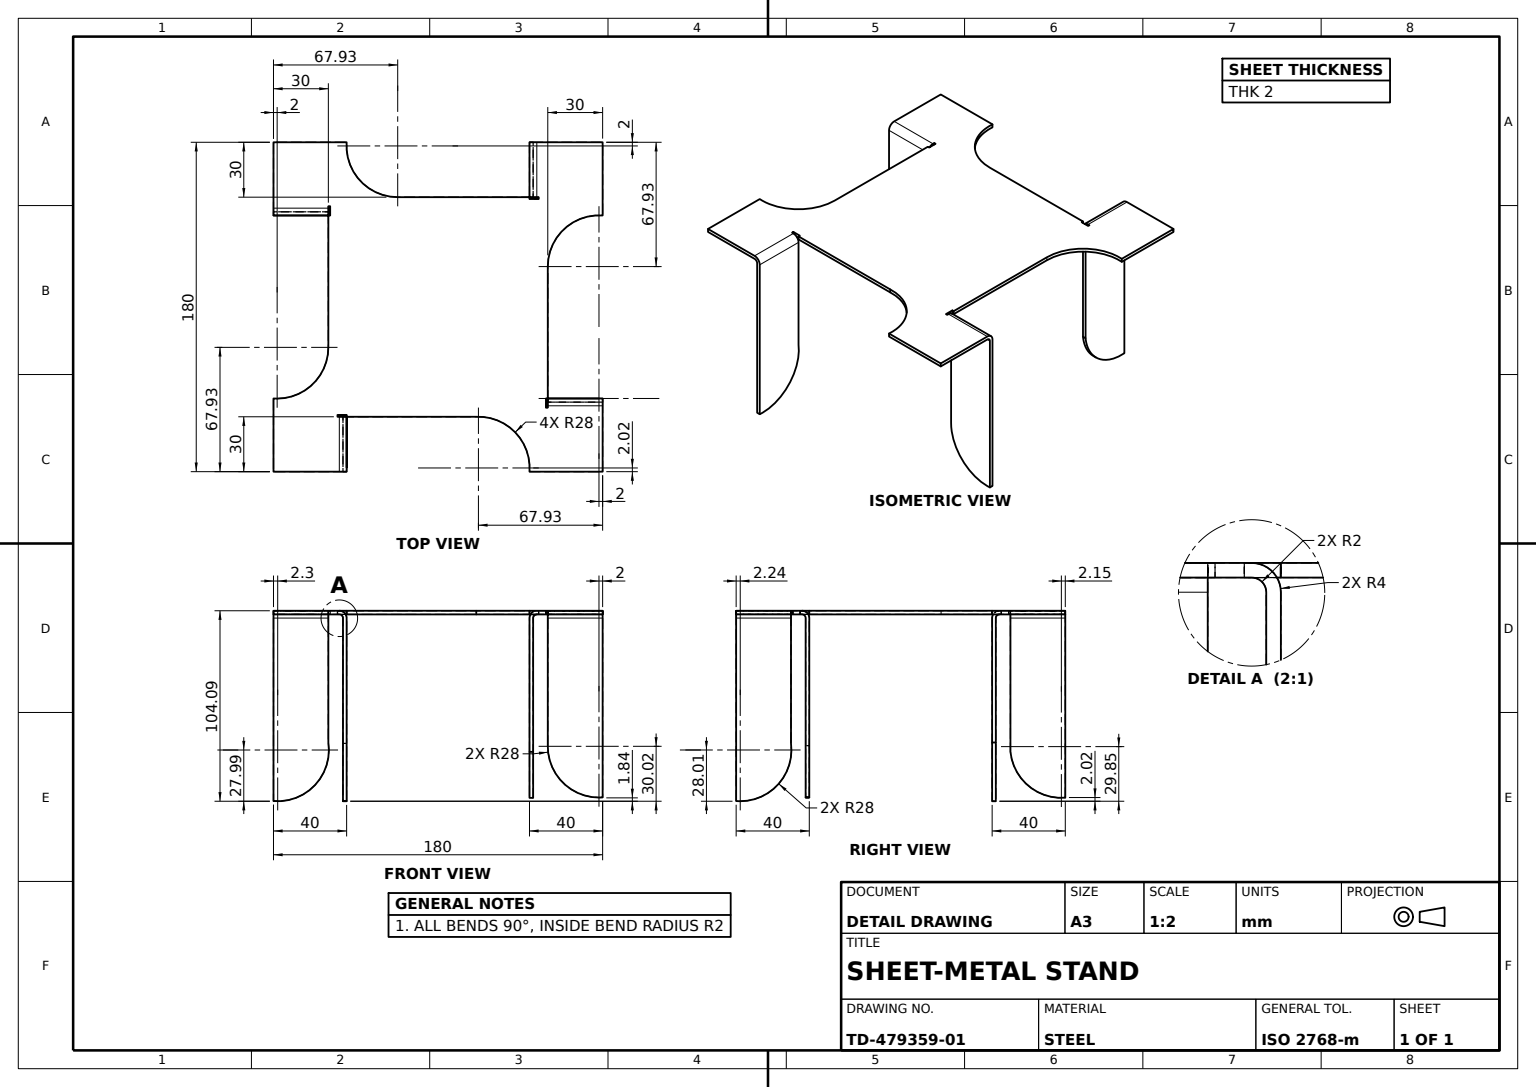
solid
v1 (60,-2,-22.07152)
v2 (60,0,-22.07152)
e1 v1 v2 LINE
v3 (60,0,50)
e2 v3 v2 LINE
v4 (60,-2,50)
e3 v4 v3 LINE
e4 v4 v1 LINE
face PLANE(AX(P(60,-2,50),D(1,0,0),D(0,0,-1))) [e1 -e2 -e3 e4]
v5 (50,0,-59)
v6 (55,0,-59)
e5 v5 v6 LINE
v7 (55,-2,-59)
e6 v7 v6 LINE
v8 (50,-2,-59)
e7 v7 v8 LINE
e8 v8 v5 LINE
face PLANE(AX(P(55,-2,-59),D(0,0,-1),D(0,1,0))) [e5 -e6 e7 e8]
v9 (-60,-2,-54)
v10 (-60,-2,-55)
e9 v9 v10 LINE
v11 (-60,0,-55)
e10 v10 v11 LINE
v12 (-60,0,-54)
e11 v11 v12 LINE
e12 v9 v12 LINE
face PLANE(AX(P(-60,-2,-54),D(1,0,0),D(0,0,-1))) [e9 e10 e11 -e12]
v13 (-54,0,60)
v14 (-50,-4,60)
e13 v13 v14 CIRCLE(AX(P(-54,-4,60),D(0,0,-1),D(1,0,0)),4)
v15 (-54,0,90)
e14 v15 v13 LINE
v16 (-50,-4,90)
e15 v16 v15 CIRCLE(AX(P(-54,-4,90),D(0,0,1),D(1,0,0)),4)
e16 v16 v14 LINE
face CYL(AX(P(-54,-4,90),D(0,0,1),D(1,0,0)),4) [-e13 -e14 -e15 e16]
v17 (-60,-2,22.07152)
v18 (-60,0,22.07152)
e17 v17 v18 LINE
v19 (-60,0,-50)
e18 v19 v18 LINE
v20 (-60,-2,-50)
e19 v20 v19 LINE
e20 v20 v17 LINE
face PLANE(AX(P(-60,-2,-50),D(-1,0,0),D(0,0,1))) [e17 -e18 -e19 e20]
v21 (-60,-4,-52)
v22 (-90,-4,-52)
e21 v21 v22 LINE
v23 (-90,-2,-54)
e22 v22 v23 CIRCLE(AX(P(-90,-4,-54),D(-1,0,0),D(0,0,1)),2)
e23 v23 v9 LINE
e24 v9 v21 CIRCLE(AX(P(-60,-4,-54),D(1,0,0),D(0,0,1)),2)
face CYL(AX(P(-90,-4,-54),D(-1,0,0),D(0,0,1)),2) rev [e21 e22 e23 e24]
v24 (-59,-2,-50)
e25 v24 v20 LINE
v25 (-59,0,-50)
e26 v19 v25 LINE
e27 v24 v25 LINE
face PLANE(AX(P(-59,-2,-50),D(0,0,-1),D(0,1,0))) [e25 e19 e26 -e27]
v26 (-50,-2,59)
v27 (-50,0,59)
e28 v26 v27 LINE
v28 (-50,-2,60)
e29 v26 v28 LINE
v29 (-50,0,60)
e30 v28 v29 LINE
e31 v29 v27 LINE
face PLANE(AX(P(-50,-2,59),D(-1,0,0),D(0,0,1))) [-e28 e29 e30 e31]
v30 (-52,-4,90)
e32 v30 v16 LINE
v31 (-54,-2,90)
e33 v31 v15 LINE
e34 v30 v31 CIRCLE(AX(P(-54,-4,90),D(0,0,1),D(1,0,0)),2)
face PLANE(AX(P(-54,-4,90),D(0,0,-1),D(-1,0,0))) rev [e32 e15 -e33 -e34]
v32 (-50,-104.089349,87.76493)
v33 (-52,-104.089349,87.76493)
e35 v32 v33 LINE
v34 (-50,-104,90)
e36 v34 v32 CIRCLE(AX(P(-50,-76.089349,87.76493),D(1,0,0),D(0,-1,0)),28)
v35 (-52,-104,90)
e37 v34 v35 LINE
e38 v35 v33 CIRCLE(AX(P(-52,-76.089349,87.76493),D(1,0,0),D(0,-1,0)),28)
face CYL(AX(P(-50,-76.089349,87.76493),D(-1,0,0),D(0,-1,0)),28) [-e35 -e36 e37 e38]
v36 (54,-2,-90)
v37 (54,0,-90)
e39 v36 v37 LINE
v38 (90,0,-90)
e40 v38 v37 LINE
v39 (90,-2,-90)
e41 v39 v38 LINE
e42 v39 v36 LINE
face PLANE(AX(P(50,-2,-90),D(0,0,-1),D(-1,0,0))) [e39 -e40 -e41 e42]
v40 (90,-2,-50)
e43 v1 v40 CIRCLE(AX(P(88,-2,-22.07152),D(0,-1,0),D(0,0,-1)),28)
v41 (90,0,-50)
e44 v40 v41 LINE
e45 v2 v41 CIRCLE(AX(P(88,0,-22.07152),D(0,-1,0),D(0,0,-1)),28)
face CYL(AX(P(88,-2,-22.07152),D(0,1,0),D(0,0,1)),28) rev [-e1 e43 e44 -e45]
v42 (-90,-104,-52)
v43 (-60,-72.002967,-52)
e46 v42 v43 CIRCLE(AX(P(-87.699422,-76.094672,-52),D(0,0,1),D(0,1,0)),28)
e47 v22 v42 LINE
e48 v43 v21 LINE
face PLANE(AX(P(-87.699422,-76.094672,-52),D(0,0,-1),D(0,1,0))) [-e46 -e47 -e21 -e48]
v44 (-90,-2,50)
v45 (-90,0,50)
e49 v44 v45 LINE
v46 (-90,-2,90)
e50 v44 v46 LINE
v47 (-90,0,90)
e51 v46 v47 LINE
e52 v45 v47 LINE
face PLANE(AX(P(-90,-2,90),D(-1,0,0),D(0,0,1))) [-e49 e50 e51 -e52]
v48 (90,-4,50)
v49 (60,-4,50)
e53 v48 v49 LINE
v50 (90,-102,50)
e54 v48 v50 LINE
v51 (87.997837,-102.071675,50)
e55 v50 v51 CIRCLE(AX(P(87.997837,-74.071675,50),D(0,0,-1),D(0,-1,0)),28)
v52 (60,-73.723608,50)
e56 v51 v52 CIRCLE(AX(P(87.997837,-74.071675,50),D(0,0,-1),D(0,-1,0)),28)
e57 v52 v49 LINE
face PLANE(AX(P(87.997837,-74.071675,50),D(0,0,1),D(0,-1,0))) rev [-e53 e54 e55 e56 e57]
v53 (90,0,90)
v54 (90,0,54)
e58 v53 v54 LINE
v55 (90,-2,90)
e59 v55 v53 LINE
v56 (90,-2,54)
e60 v55 v56 LINE
e61 v56 v54 LINE
face PLANE(AX(P(90,-2,90),D(1,0,0),D(0,0,-1))) [-e58 -e59 e60 e61]
v57 (-50,-72.46876,60)
e62 v32 v57 CIRCLE(AX(P(-50,-76.089349,87.76493),D(1,0,0),D(0,-1,0)),28)
e63 v57 v14 LINE
e64 v16 v34 LINE
face PLANE(AX(P(-50,-76.089349,87.76493),D(-1,0,0),D(0,-1,0))) rev [e62 e63 -e16 e64 e36]
e65 v47 v15 LINE
e66 v46 v31 LINE
face PLANE(AX(P(-90,-2,90),D(0,0,1),D(1,0,0))) [-e65 -e51 e66 e33]
v58 (50,-77.10989,-60)
v59 (50,-4,-60)
e67 v58 v59 LINE
v60 (52,-77.10989,-60)
e68 v58 v60 LINE
v61 (52,-4,-60)
e69 v60 v61 LINE
e70 v61 v59 LINE
face PLANE(AX(P(50,-2,-60),D(0,0,-1),D(-1,0,0))) rev [-e67 e68 e69 e70]
v62 (60,0,54)
e71 v62 v49 CIRCLE(AX(P(60,-4,54),D(-1,0,0),D(0,0,-1)),4)
v63 (60,-4,52)
e72 v63 v49 LINE
v64 (60,-2,54)
e73 v64 v63 CIRCLE(AX(P(60,-4,54),D(-1,0,0),D(0,0,-1)),2)
e74 v64 v62 LINE
face PLANE(AX(P(60,-4,54),D(-1,0,0),D(0,0,1))) [e71 -e72 -e73 e74]
v65 (90,-4,52)
e75 v65 v48 LINE
e76 v48 v54 CIRCLE(AX(P(90,-4,54),D(1,0,0),D(0,0,-1)),4)
e77 v65 v56 CIRCLE(AX(P(90,-4,54),D(1,0,0),D(0,0,-1)),2)
face PLANE(AX(P(90,-4,54),D(-1,0,0),D(0,0,1))) rev [e75 e76 -e61 -e77]
v66 (90,-102,52)
v67 (87.997837,-102.071675,52)
e78 v66 v67 CIRCLE(AX(P(87.997837,-74.071675,52),D(0,0,-1),D(0,-1,0)),28)
e79 v51 v67 LINE
e80 v50 v66 LINE
face CYL(AX(P(87.997837,-74.071675,50),D(0,0,1),D(0,-1,0)),28) [e78 -e79 -e55 e80]
v68 (52,-4,-90)
e81 v61 v68 LINE
e82 v68 v36 CIRCLE(AX(P(54,-4,-90),D(0,0,-1),D(-1,0,0)),2)
v69 (54,-2,-60)
e83 v36 v69 LINE
e84 v69 v61 CIRCLE(AX(P(54,-4,-60),D(0,0,1),D(-1,0,0)),2)
face CYL(AX(P(54,-4,-90),D(0,0,-1),D(-1,0,0)),2) rev [e81 e82 e83 e84]
v70 (-60,-72.002967,-50)
e85 v70 v43 LINE
v71 (-60,-4,-50)
e86 v21 v71 LINE
e87 v70 v71 LINE
face PLANE(AX(P(-60,-2,-50),D(-1,0,0),D(0,0,1))) rev [e85 e48 e86 -e87]
v72 (50,-4,-90)
e88 v72 v37 CIRCLE(AX(P(54,-4,-90),D(0,0,-1),D(-1,0,0)),4)
e89 v72 v59 LINE
v73 (54,0,-60)
e90 v73 v59 CIRCLE(AX(P(54,-4,-60),D(0,0,1),D(-1,0,0)),4)
e91 v37 v73 LINE
face CYL(AX(P(54,-4,-90),D(0,0,-1),D(-1,0,0)),4) [-e88 e89 -e90 -e91]
v74 (55,-2,-60)
e92 v74 v7 LINE
v75 (55,0,-60)
e93 v6 v75 LINE
e94 v74 v75 LINE
face PLANE(AX(P(55,-2,-60),D(-1,0,0),D(0,0,1))) [e92 e6 e93 -e94]
e95 v69 v74 LINE
e96 v75 v73 LINE
e97 v69 v73 LINE
face PLANE(AX(P(54,-2,-60),D(0,0,1),D(0,-1,0))) [e95 e94 e96 -e97]
e98 v30 v35 LINE
v76 (-52,-4,60)
e99 v76 v30 LINE
v77 (-52,-72.46876,60)
e100 v77 v76 LINE
e101 v33 v77 CIRCLE(AX(P(-52,-76.089349,87.76493),D(1,0,0),D(0,-1,0)),28)
face PLANE(AX(P(-52,-76.089349,87.76493),D(-1,0,0),D(0,-1,0))) [-e98 -e99 -e100 -e101 -e38]
v78 (-55,-2,60)
v79 (-55,-2,59)
e102 v78 v79 LINE
v80 (-55,0,59)
e103 v79 v80 LINE
v81 (-55,0,60)
e104 v80 v81 LINE
e105 v78 v81 LINE
face PLANE(AX(P(-55,-2,60),D(1,0,0),D(0,0,-1))) [e102 e103 e104 -e105]
face PLANE(AX(P(-50,-104,90),D(0,0,-1),D(0,1,0))) rev [-e64 -e32 e98 -e37]
v82 (-59,-2,-55)
e106 v10 v82 LINE
v83 (-59,0,-55)
e107 v82 v83 LINE
e108 v83 v11 LINE
face PLANE(AX(P(-60,-2,-55),D(0,0,1),D(0,-1,0))) [e106 e107 e108 -e10]
v84 (52,-102.164826,-90)
e109 v84 v60 CIRCLE(AX(P(52,-74.247241,-87.853281),D(-1,0,0),D(0,1,0)),28)
e110 v68 v84 LINE
face PLANE(AX(P(52,-74.247241,-87.853281),D(1,0,0),D(0,1,0))) [-e69 -e109 -e110 -e81]
v85 (59,0,50)
e111 v3 v85 LINE
v86 (59,-2,50)
e112 v86 v85 LINE
e113 v86 v4 LINE
face PLANE(AX(P(59,-2,50),D(0,0,1),D(0,-1,0))) [e111 -e112 e113 e3]
v87 (-54,-2,60)
e114 v87 v76 CIRCLE(AX(P(-54,-4,60),D(0,0,-1),D(1,0,0)),2)
e115 v31 v87 LINE
face CYL(AX(P(-54,-4,90),D(0,0,1),D(1,0,0)),2) rev [e114 e99 e34 e115]
e116 v76 v14 LINE
e117 v87 v13 LINE
face PLANE(AX(P(-54,-4,60),D(0,0,-1),D(-1,0,0))) [-e116 -e114 e117 e13]
e118 v82 v24 LINE
e119 v25 v83 LINE
face PLANE(AX(P(-59,-2,-55),D(-1,0,0),D(0,0,1))) [e118 e27 e119 -e107]
e120 v57 v77 LINE
face CYL(AX(P(-50,-76.089349,87.76493),D(-1,0,0),D(0,-1,0)),28) [e35 e101 -e120 -e62]
v88 (-90,-4,-50)
v89 (-90,-104,-50)
e121 v88 v89 LINE
e122 v22 v88 LINE
e123 v89 v42 LINE
face PLANE(AX(P(-90,-104,-50),D(1,0,0),D(0,1,0))) rev [-e121 -e122 e47 -e123]
v90 (50,0,90)
e124 v90 v53 LINE
v91 (50,-2,90)
e125 v91 v90 LINE
e126 v91 v55 LINE
face PLANE(AX(P(90,-2,90),D(0,0,1),D(1,0,0))) [-e124 -e125 e126 e59]
v92 (60,-2,55)
v93 (60,0,55)
e127 v92 v93 LINE
v94 (59,-2,55)
e128 v92 v94 LINE
v95 (59,0,55)
e129 v94 v95 LINE
e130 v95 v93 LINE
face PLANE(AX(P(60,-2,55),D(0,0,-1),D(0,1,0))) [-e127 e128 e129 e130]
v96 (20.89418,0,60)
e131 v96 v90 CIRCLE(AX(P(22.07331,0,87.975161),D(0,-1,0),D(0,0,-1)),28)
v97 (20.89418,-2,60)
e132 v97 v96 LINE
e133 v97 v91 CIRCLE(AX(P(22.07331,-2,87.975161),D(0,-1,0),D(0,0,-1)),28)
face CYL(AX(P(22.07331,-2,87.975161),D(0,1,0),D(0,0,1)),28) rev [-e131 -e132 e133 e125]
face PLANE(AX(P(-50,-2,60),D(0,0,1),D(1,0,0))) rev [e116 -e63 e120 e100]
e134 v40 v39 LINE
e135 v94 v86 LINE
e136 v64 v92 LINE
e137 v56 v64 LINE
e138 v28 v97 LINE
e139 v79 v26 LINE
e140 v87 v78 LINE
v98 (-88,-2,50.07152)
e141 v98 v44 CIRCLE(AX(P(-88,-2,22.07152),D(0,-1,0),D(0,0,-1)),28)
e142 v17 v98 CIRCLE(AX(P(-88,-2,22.07152),D(0,-1,0),D(0,0,-1)),28)
v99 (-90,-2,-90)
e143 v99 v23 LINE
v100 (-50,-2,-90)
e144 v100 v99 LINE
v101 (-22.07152,-2,-60)
e145 v101 v100 CIRCLE(AX(P(-22.07152,-2,-88),D(0,-1,0),D(0,0,-1)),28)
v102 (50,-2,-60)
e146 v102 v101 LINE
e147 v8 v102 LINE
face PLANE(AX(P(88,-2,-22.07152),D(0,-1,0),D(0,0,-1))) [-e42 -e134 -e43 -e4 -e113 -e135 -e128 -e136 -e137 -e60 -e126 -e133 -e138 -e29 -e139 -e102 -e140 -e115 -e66 -e50 -e141 -e142 -e20 -e25 -e118 -e106 -e9 -e23 -e143 -e144 -e145 -e146 -e147 -e7 -e92 -e95 -e83]
v103 (-50,0,-90)
e148 v100 v103 LINE
v104 (-90,0,-90)
e149 v99 v104 LINE
e150 v103 v104 LINE
face PLANE(AX(P(-90,-2,-90),D(0,0,-1),D(-1,0,0))) [-e148 e144 e149 -e150]
e151 v41 v38 LINE
face PLANE(AX(P(90,-2,-50),D(1,0,0),D(0,0,-1))) [e41 -e151 -e44 e134]
v105 (50,-102.164826,-90)
e152 v105 v58 CIRCLE(AX(P(50,-74.247241,-87.853281),D(-1,0,0),D(0,1,0)),28)
e153 v105 v84 LINE
face CYL(AX(P(50,-74.247241,-87.853281),D(1,0,0),D(0,1,0)),28) [e109 -e68 -e152 e153]
e154 v27 v80 LINE
face PLANE(AX(P(-55,-2,59),D(0,0,1),D(0,-1,0))) [e154 -e103 e139 e28]
e155 v72 v105 LINE
face PLANE(AX(P(50,-74.247241,-87.853281),D(1,0,0),D(0,1,0))) rev [-e89 e155 e152 e67]
v106 (-90,0,-54)
e156 v88 v106 CIRCLE(AX(P(-90,-4,-54),D(-1,0,0),D(0,0,1)),4)
e157 v23 v106 LINE
face PLANE(AX(P(-90,-4,-54),D(1,0,0),D(0,0,-1))) rev [e122 e156 -e157 -e22]
v107 (60,-73.723608,52)
e158 v52 v107 LINE
e159 v107 v63 LINE
face PLANE(AX(P(60,-2,50),D(1,0,0),D(0,0,-1))) rev [-e57 e158 e159 e72]
e160 v65 v66 LINE
face PLANE(AX(P(90,-102,50),D(-1,0,0),D(0,0,1))) rev [-e80 -e54 -e75 e160]
e161 v88 v71 LINE
e162 v89 v70 CIRCLE(AX(P(-87.699422,-76.094672,-50),D(0,0,1),D(0,1,0)),28)
face PLANE(AX(P(-87.699422,-76.094672,-50),D(0,0,-1),D(0,1,0))) rev [-e161 e121 e162 e87]
face CYL(AX(P(-87.699422,-76.094672,-50),D(0,0,-1),D(0,1,0)),28) [-e85 -e162 e123 e46]
e163 v67 v107 CIRCLE(AX(P(87.997837,-74.071675,52),D(0,0,-1),D(0,-1,0)),28)
face CYL(AX(P(87.997837,-74.071675,50),D(0,0,1),D(0,-1,0)),28) [e163 -e158 -e56 e79]
e164 v68 v72 LINE
face PLANE(AX(P(54,-4,-90),D(0,0,1),D(1,0,0))) rev [e164 e88 -e39 -e82]
v108 (50,0,-60)
e165 v102 v108 LINE
e166 v108 v5 LINE
face PLANE(AX(P(50,-2,-59),D(1,0,0),D(0,0,-1))) [e165 e166 -e8 e147]
v109 (-22.07152,0,-60)
e167 v101 v109 LINE
e168 v109 v103 CIRCLE(AX(P(-22.07152,0,-88),D(0,-1,0),D(0,0,-1)),28)
face CYL(AX(P(-22.07152,-2,-88),D(0,1,0),D(0,0,1)),28) rev [-e167 e145 e148 -e168]
e169 v63 v65 LINE
face PLANE(AX(P(87.997837,-74.071675,52),D(0,0,1),D(0,-1,0))) [-e78 -e160 -e169 -e159 -e163]
e170 v93 v62 LINE
face PLANE(AX(P(60,-2,54),D(-1,0,0),D(0,0,1))) [e127 e170 -e74 e136]
face PLANE(AX(P(50,-102.164826,-90),D(0,0,1),D(1,0,0))) rev [-e153 -e155 -e164 e110]
e171 v81 v13 LINE
face PLANE(AX(P(-54,-2,60),D(0,0,-1),D(0,1,0))) [e171 -e117 e140 e105]
e172 v106 v12 LINE
e173 v12 v71 CIRCLE(AX(P(-60,-4,-54),D(1,0,0),D(0,0,1)),4)
face CYL(AX(P(-90,-4,-54),D(-1,0,0),D(0,0,1)),4) [-e172 -e156 e161 -e173]
e174 v85 v95 LINE
face PLANE(AX(P(59,-2,55),D(1,0,0),D(0,0,-1))) [-e129 e135 e112 e174]
v110 (-88,0,50.07152)
e175 v98 v110 LINE
e176 v18 v110 CIRCLE(AX(P(-88,0,22.07152),D(0,-1,0),D(0,0,-1)),28)
face CYL(AX(P(-88,-2,22.07152),D(0,1,0),D(0,0,1)),28) rev [e142 e175 -e176 -e17]
face CYL(AX(P(90,-4,54),D(1,0,0),D(0,0,-1)),2) rev [e77 e137 e73 e169]
e177 v108 v109 LINE
face PLANE(AX(P(50,-2,-60),D(0,0,-1),D(-1,0,0))) [e146 e167 -e177 -e165]
e178 v104 v106 LINE
face PLANE(AX(P(-90,-2,-50),D(-1,0,0),D(0,0,1))) [e157 -e178 -e149 e143]
face PLANE(AX(P(-60,-4,-54),D(1,0,0),D(0,0,-1))) [e173 -e86 -e24 e12]
e179 v110 v45 CIRCLE(AX(P(-88,0,22.07152),D(0,-1,0),D(0,0,-1)),28)
face CYL(AX(P(-88,-2,22.07152),D(0,1,0),D(0,0,1)),28) rev [e141 e49 -e179 -e175]
e180 v54 v62 LINE
face CYL(AX(P(90,-4,54),D(1,0,0),D(0,0,-1)),4) [-e71 -e180 -e76 e53]
e181 v29 v96 LINE
face PLANE(AX(P(-50,-2,60),D(0,0,1),D(1,0,0))) [e132 -e181 -e30 e138]
face PLANE(AX(P(88,0,-22.07152),D(0,-1,0),D(0,0,-1))) rev [e168 e150 e178 e172 -e11 -e108 -e119 -e26 e18 e176 e179 e52 e65 e14 -e171 -e104 -e154 -e31 e181 e131 e124 e58 e180 -e170 -e130 -e174 -e111 e2 e45 e151 e40 e91 -e96 -e93 -e5 -e166 e177]
face PLANE(AX(P(54,-4,-60),D(0,0,1),D(1,0,0))) [-e84 e97 e90 -e70]
